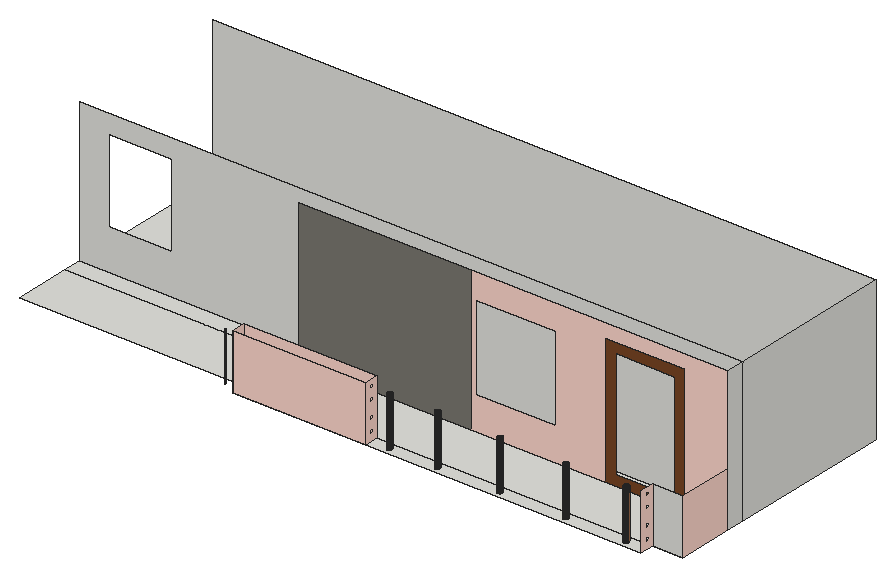
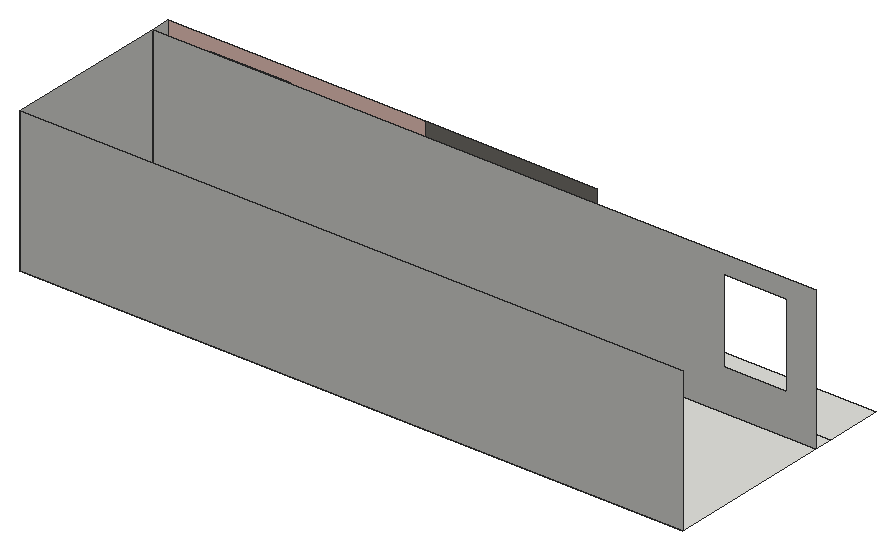
# SketchUp Ruby script. Lengths in inches.
U = 1.inch
M = Sketchup.active_model
def pt(a) = Geom::Point3d.new(a.map { |v| v * U })
def face(e, loops, mat)
  f = e.add_face(loops[0].map { |a| pt(a) })
  loops[1..].each { |l| e.add_face(l.map { |a| pt(a) }).erase! }
  f.material = f.back_material = mat if mat
  f
end
# faces: each face lists its corners as indices into pts; further lists are holes
def faces(e, pts, list, mat = nil) = list.each { |f| face(e, (f[0].is_a?(Array) ? f : [f]).map { |l| l.map { |i| pts[i] } }, mat) }
# xy, xz, yz: faces in a plane at the given z, y or x. An outline is a flat list of corners, or four numbers for a rectangle; further outlines are holes
def ring(l) = l.size == 4 ? [[l[0], l[1]], [l[2], l[1]], [l[2], l[3]], [l[0], l[3]]] : l.each_slice(2).to_a
def flat(e, list, mat, &to3) = list.each { |f| face(e, (f[0].is_a?(Array) ? f : [f]).map { |l| ring(l).map { |u, v| to3.(u, v) } }, mat) }
def xy(e, z, list, mat = nil) = flat(e, list, mat) { |x, y| [x, y, z] }
def xz(e, y, list, mat = nil) = flat(e, list, mat) { |x, z| [x, y, z] }
def yz(e, x, list, mat = nil) = flat(e, list, mat) { |y, z| [x, y, z] }
def lines(e, pts, list) = list.each { |a, b| e.add_line(pt(pts[a]), pt(pts[b])) }
# prism: a flat outline (further loops are holes) pulled along v
def prism(e, loops, v, mat = nil)
  f = face(e, loops, mat); d = Geom::Vector3d.new(v.map { |x| x * U })
  f.pushpull(f.normal.samedirection?(d) ? d.length : -d.length)
end
def box(e, o, s, mat = nil) = prism(e, [[o, [o[0] + s[0], o[1], o[2]], [o[0] + s[0], o[1] + s[1], o[2]], [o[0], o[1] + s[1], o[2]]]], [0, 0, s[2]], mat)
def at(x, y, z, deg = 0) = Geom::Transformation.translation(pt([x, y, z])) * Geom::Transformation.rotation(ORIGIN, Z_AXIS, deg.degrees)
def axes(o, x, y, z) = Geom::Transformation.new([*x, 0, *y, 0, *z, 0, *pt(o).to_a, 1])
def part(name) = M.definitions.add(name)
# library, detail: a bought-in or finely detailed component or shape, given as its bounding box
def library(name, o, s) = part(name).tap { |d| box(d.entities, o, s) }
def detail(e, o, s) = box(e.add_group.entities, o, s)
def put(e, d, t, mat = nil) = e.add_instance(d, t).tap { |i| i.material = mat if mat }
def group(e, t, mat = nil) = e.add_group.tap { |g| g.transformation = t; g.material = mat if mat }.entities
root = M.entities
M.materials.add("[Color B01]").color = [255, 216, 204]
M.materials.add("[Rough Square Concrete Block]").color = [123, 120, 113]
M.materials.add("[Wood Veneer 01]1").color = [120, 70, 37]
M.materials.add("[Wood Veneer 02]").color = [190, 128, 91]
xy(root,1956.4375,[[1053.15,267.5625,1631.4,328.8],[[1631.4,267.5625,2829.41,328.8],[1711.75,285.86,1709,286.22,1706.4375,287.28,1704.24,288.97,1702.55,291.17,1701.49,293.73,1701.125,296.48,1701.49,299.23,1702.55,301.79,1704.24,303.99,1706.4375,305.68,1709,306.74,1711.75,307.11,1714.5,306.74,1717.0625,305.68,1719.26,303.99,1720.95,301.79,1722.01,299.23,1722.375,296.48,1722.01,293.73,1720.95,291.17,1719.26,288.97,1717.0625,287.28,1714.5,286.22],[2741.25,285.86,2738.5,286.22,2735.9375,287.28,2733.74,288.97,2732.05,291.17,2730.99,293.73,2730.625,296.48,2730.99,299.23,2732.05,301.79,2733.74,303.99,2735.9375,305.68,2738.5,306.74,2741.25,307.11,2744,306.74,2746.5625,305.68,2748.76,303.99,2750.45,301.79,2751.51,299.23,2751.875,296.48,2751.51,293.73,2750.45,291.17,2748.76,288.97,2746.5625,287.28,2744,286.22],[1920.9375,285.86,1918.1875,286.22,1915.625,287.28,1913.42,288.97,1911.74,291.17,1910.67,293.73,1910.3125,296.48,1910.67,299.23,1911.74,301.79,1913.42,303.99,1915.625,305.68,1918.1875,306.74,1920.9375,307.11,1923.6875,306.74,1926.25,305.68,1928.45,303.99,1930.14,301.79,1931.2,299.23,1931.5625,296.48,1931.2,293.73,1930.14,291.17,1928.45,288.97,1926.25,287.28,1923.6875,286.22],[2479.625,285.86,2476.875,286.22,2474.3125,287.28,2472.11,288.97,2470.42,291.17,2469.36,293.73,2469,296.48,2469.36,299.23,2470.42,301.79,2472.11,303.99,2474.3125,305.68,2476.875,306.74,2479.625,307.11,2482.375,306.74,2484.9375,305.68,2487.14,303.99,2488.83,301.79,2489.89,299.23,2490.25,296.48,2489.89,293.73,2488.83,291.17,2487.14,288.97,2484.9375,287.28,2482.375,286.22],[2192.5,285.86,2189.75,286.22,2187.1875,287.28,2184.99,288.97,2183.3,291.17,2182.24,293.73,2181.875,296.48,2182.24,299.23,2183.3,301.79,2184.99,303.99,2187.1875,305.68,2189.75,306.74,2192.5,307.11,2195.25,306.74,2197.8125,305.68,2200.01,303.99,2201.7,301.79,2202.76,299.23,2203.125,296.48,2202.76,293.73,2201.7,291.17,2200.01,288.97,2197.8125,287.28,2195.25,286.22]],[1711.75,285.86,1709,286.22,1706.4375,287.28,1704.24,288.97,1702.55,291.17,1701.49,293.73,1701.125,296.48,1701.49,299.23,1702.55,301.79,1704.24,303.99,1706.4375,305.68,1709,306.74,1711.75,307.11,1714.5,306.74,1717.0625,305.68,1719.26,303.99,1720.95,301.79,1722.01,299.23,1722.375,296.48,1722.01,293.73,1720.95,291.17,1719.26,288.97,1717.0625,287.28,1714.5,286.22],[1920.9375,285.86,1918.1875,286.22,1915.625,287.28,1913.42,288.97,1911.74,291.17,1910.67,293.73,1910.3125,296.48,1910.67,299.23,1911.74,301.79,1913.42,303.99,1915.625,305.68,1918.1875,306.74,1920.9375,307.11,1923.6875,306.74,1926.25,305.68,1928.45,303.99,1930.14,301.79,1931.2,299.23,1931.5625,296.48,1931.2,293.73,1930.14,291.17,1928.45,288.97,1926.25,287.28,1923.6875,286.22],[2192.5,285.86,2189.75,286.22,2187.1875,287.28,2184.99,288.97,2183.3,291.17,2182.24,293.73,2181.875,296.48,2182.24,299.23,2183.3,301.79,2184.99,303.99,2187.1875,305.68,2189.75,306.74,2192.5,307.11,2195.25,306.74,2197.8125,305.68,2200.01,303.99,2201.7,301.79,2202.76,299.23,2203.125,296.48,2202.76,293.73,2201.7,291.17,2200.01,288.97,2197.8125,287.28,2195.25,286.22],
  [2479.625,285.86,2476.875,286.22,2474.3125,287.28,2472.11,288.97,2470.42,291.17,2469.36,293.73,2469,296.48,2469.36,299.23,2470.42,301.79,2472.11,303.99,2474.3125,305.68,2476.875,306.74,2479.625,307.11,2482.375,306.74,2484.9375,305.68,2487.14,303.99,2488.83,301.79,2489.89,299.23,2490.25,296.48,2489.89,293.73,2488.83,291.17,2487.14,288.97,2484.9375,287.28,2482.375,286.22],[2741.25,285.86,2738.5,286.22,2735.9375,287.28,2733.74,288.97,2732.05,291.17,2730.99,293.73,2730.625,296.48,2730.99,299.23,2732.05,301.79,2733.74,303.99,2735.9375,305.68,2738.5,306.74,2741.25,307.11,2744,306.74,2746.5625,305.68,2748.76,303.99,2750.45,301.79,2751.51,299.23,2751.875,296.48,2751.51,293.73,2750.45,291.17,2748.76,288.97,2746.5625,287.28,2744,286.22],[77.93,328.8,2962.22,571.9],[77.93,571.9,2962.22,653.97],[77.93,653.97,2962.22,1377.24]])
xz(root,267.5625,[[1053.15,1956.4375,1631.4,2195.8125]],"[Color B01]")
xz(root,328.8,[[2829.41,1956.4375,2962.22,2195.8125]])
xz(root,328.8,[[1053.15,1956.4375,1631.4,2195.8125]],"[Color B01]")
xz(root,571.9,[[[1845.89,1956.4375,2429.34,1956.4375,2429.34,2519.61,2777.4,2519.61,2777.4,1956.4375,2962.22,1956.4375,2962.22,2577.9375,1845.89,2577.9375],[1867.29,2101.11,2212.79,2469.24]]],"[Color B01]")
xz(root,571.9,[[1096.47,1956.4375,1845.89,2577.9375]],"[Rough Square Concrete Block]")
xz(root,571.9,[[[2429.34,1956.4375,2777.4,2519.61],[2473.97,2001.07,2732.77,2474.99]]],"[Wood Veneer 01]1")
xz(root,653.97,[[[77.93,1956.4375,2962.22,2577.9375],[206.78,2135.23,480.91,2496.04]]])
xz(root,1377.24,[[77.93,1956.4375,2962.22,2577.9375]])
yz(root,1053.15,[[[267.5625,1956.4375,328.8,2195.8125],[300.84,2164.31,302.34,2164.51,303.74,2165.09,304.95,2166.01,305.87,2167.21,306.45,2168.62,306.65,2170.12,306.45,2171.625,305.87,2173.03,304.95,2174.23,303.74,2175.15,302.34,2175.73,300.84,2175.93,299.33,2175.73,297.93,2175.15,296.73,2174.23,295.8,2173.03,295.22,2171.625,295.02,2170.12,295.22,2168.62,295.8,2167.21,296.73,2166.01,297.93,2165.09,299.33,2164.51],[300.84,1977.93,302.34,1978.13,303.74,1978.71,304.95,1979.63,305.87,1980.84,306.45,1982.24,306.65,1983.74,306.45,1985.25,305.87,1986.65,304.95,1987.85,303.74,1988.78,302.34,1989.36,300.84,1989.56,299.33,1989.36,297.93,1988.78,296.73,1987.85,295.8,1986.65,295.22,1985.25,295.02,1983.74,295.22,1982.24,295.8,1980.84,296.73,1979.63,297.93,1978.71,299.33,1978.13],[300.84,2119.12,302.34,2119.32,303.74,2119.9,304.95,2120.82,305.87,2122.03,306.45,2123.43,306.65,2124.93,306.45,2126.4375,305.87,2127.84,304.95,2129.04,303.74,2129.97,302.34,2130.55,300.84,2130.74,299.33,2130.55,297.93,2129.97,296.73,2129.04,295.8,2127.84,295.22,2126.4375,295.02,2124.93,295.22,2123.43,295.8,2122.03,296.73,2120.82,297.93,2119.9,299.33,2119.32],[300.84,2017.49,302.34,2017.69,303.74,2018.27,304.95,2019.2,305.87,2020.4,306.45,2021.8,306.65,2023.31,306.45,2024.8125,305.87,2026.21,304.95,2027.42,303.74,2028.34,302.34,2028.92,300.84,2029.12,299.33,2028.92,297.93,2028.34,296.73,2027.42,295.8,2026.21,295.22,2024.8125,295.02,2023.31,295.22,2021.8,295.8,2020.4,296.73,2019.2,297.93,2018.27,299.33,2017.69],[300.84,2076.99,302.34,2077.19,303.74,2077.77,304.95,2078.7,305.87,2079.9,306.45,2081.3,306.65,2082.81,306.45,2084.3125,305.87,2085.71,304.95,2086.92,303.74,2087.84,302.34,2088.42,300.84,2088.62,299.33,2088.42,297.93,2087.84,296.73,2086.92,295.8,2085.71,295.22,2084.3125,295.02,2082.81,295.22,2081.3,295.8,2079.9,296.73,2078.7,297.93,2077.77,299.33,2077.19]]],"[Color B01]")
yz(root,1631.4,[[[267.5625,1956.4375,328.8,2195.8125],[299.17,2162.9,296.83,2163.21,294.64,2164.12,292.77,2165.56,291.33,2167.43,290.42,2169.62,290.11,2171.97,290.42,2174.3125,291.33,2176.5,292.77,2178.375,294.64,2179.8125,296.83,2180.72,299.17,2181.03,301.52,2180.72,303.71,2179.8125,305.58,2178.375,307.02,2176.5,307.93,2174.3125,308.24,2171.97,307.93,2169.62,307.02,2167.43,305.58,2165.56,303.71,2164.12,301.52,2163.21],[299.17,2111.15,296.83,2111.46,294.64,2112.37,292.77,2113.81,291.33,2115.68,290.42,2117.87,290.11,2120.22,290.42,2122.5625,291.33,2124.75,292.77,2126.625,294.64,2128.0625,296.83,2128.97,299.17,2129.28,301.52,2128.97,303.71,2128.0625,305.58,2126.625,307.02,2124.75,307.93,2122.5625,308.24,2120.22,307.93,2117.87,307.02,2115.68,305.58,2113.81,303.71,2112.37,301.52,2111.46],[299.17,2040.72,296.83,2041.02,294.64,2041.93,292.77,2043.37,291.33,2045.25,290.42,2047.43,290.11,2049.78,290.42,2052.125,291.33,2054.31,292.77,2056.1875,294.64,2057.625,296.83,2058.53,299.17,2058.84,301.52,2058.53,303.71,2057.625,305.58,2056.1875,307.02,2054.31,307.93,2052.125,308.24,2049.78,307.93,2047.43,307.02,2045.25,305.58,2043.37,303.71,2041.93,301.52,2041.02],[299.17,1985.65,296.83,1985.96,294.64,1986.87,292.77,1988.31,291.33,1990.18,290.42,1992.37,290.11,1994.72,290.42,1997.0625,291.33,1999.25,292.77,2001.125,294.64,2002.5625,296.83,2003.47,299.17,2003.78,301.52,2003.47,303.71,2002.5625,305.58,2001.125,307.02,1999.25,307.93,1997.0625,308.24,1994.72,307.93,1992.37,307.02,1990.18,305.58,1988.31,303.71,1986.87,301.52,1985.96]]],"[Color B01]")
yz(root,2829.41,[[[267.5625,1956.4375,328.8,2195.8125],[299.17,2162.9,301.52,2163.21,303.71,2164.12,305.58,2165.56,307.02,2167.43,307.93,2169.62,308.24,2171.97,307.93,2174.3125,307.02,2176.5,305.58,2178.375,303.71,2179.8125,301.52,2180.72,299.17,2181.03,296.83,2180.72,294.64,2179.8125,292.77,2178.375,291.33,2176.5,290.42,2174.3125,290.11,2171.97,290.42,2169.62,291.33,2167.43,292.77,2165.56,294.64,2164.12,296.83,2163.21],[299.17,1985.65,301.52,1985.96,303.71,1986.87,305.58,1988.31,307.02,1990.18,307.93,1992.37,308.24,1994.72,307.93,1997.0625,307.02,1999.25,305.58,2001.125,303.71,2002.5625,301.52,2003.47,299.17,2003.78,296.83,2003.47,294.64,2002.5625,292.77,2001.125,291.33,1999.25,290.42,1997.0625,290.11,1994.72,290.42,1992.37,291.33,1990.18,292.77,1988.31,294.64,1986.87,296.83,1985.96],[299.17,2111.15,301.52,2111.46,303.71,2112.37,305.58,2113.81,307.02,2115.68,307.93,2117.87,308.24,2120.22,307.93,2122.5625,307.02,2124.75,305.58,2126.625,303.71,2128.0625,301.52,2128.97,299.17,2129.28,296.83,2128.97,294.64,2128.0625,292.77,2126.625,291.33,2124.75,290.42,2122.5625,290.11,2120.22,290.42,2117.87,291.33,2115.68,292.77,2113.81,294.64,2112.37,296.83,2111.46],[299.17,2040.72,301.52,2041.02,303.71,2041.93,305.58,2043.37,307.02,2045.25,307.93,2047.43,308.24,2049.78,307.93,2052.125,307.02,2054.31,305.58,2056.1875,303.71,2057.625,301.52,2058.53,299.17,2058.84,296.83,2058.53,294.64,2057.625,292.77,2056.1875,291.33,2054.31,290.42,2052.125,290.11,2049.78,290.42,2047.43,291.33,2045.25,292.77,2043.37,294.64,2041.93,296.83,2041.02]]],"[Color B01]")
yz(root,2962.22,[[571.9,1956.4375,653.97,2577.9375],[653.97,1956.4375,1377.24,2577.9375]])
yz(root,2962.22,[[328.8,1956.4375,571.9,2195.8125]],"[Color B01]")
p = [[1709,286.22,1956.4375],[1711.75,285.86,1956.4375],[1711.75,285.86,2171.4375],[1709,286.22,2171.4375],[1714.5,286.22,1956.4375],[1714.5,286.22,2171.4375],
  [1918.1875,286.22,1956.4375],[1920.9375,285.86,1956.4375],[1920.9375,285.86,2176.5],[1918.1875,286.22,2176.5],[1923.6875,286.22,1956.4375],[1923.6875,286.22,2176.5],
  [2189.75,286.22,1956.4375],[2192.5,285.86,1956.4375],[2192.5,285.86,2169.6875],[2189.75,286.22,2169.6875],[2195.25,286.22,1956.4375],[2195.25,286.22,2169.6875],
  [2476.875,286.22,1956.4375],[2479.625,285.86,1956.4375],[2479.625,285.86,2168.9375],[2476.875,286.22,2168.9375],[2482.375,286.22,1956.4375],[2482.375,286.22,2168.9375],
  [2738.5,286.22,1956.4375],[2741.25,285.86,1956.4375],[2741.25,285.86,2173.25],[2738.5,286.22,2173.25],[2744,286.22,1956.4375],[2744,286.22,2173.25],
  [1706.4375,287.28,1956.4375],[1706.4375,287.28,2171.4375],[1717.0625,287.28,1956.4375],[1717.0625,287.28,2171.4375],[1915.625,287.28,1956.4375],[1915.625,287.28,2176.5],
  [1926.25,287.28,1956.4375],[1926.25,287.28,2176.5],[2187.1875,287.28,1956.4375],[2187.1875,287.28,2169.6875],[2197.8125,287.28,1956.4375],[2197.8125,287.28,2169.6875],
  [2474.3125,287.28,1956.4375],[2474.3125,287.28,2168.9375],[2484.9375,287.28,1956.4375],[2484.9375,287.28,2168.9375],[2735.9375,287.28,1956.4375],[2735.9375,287.28,2173.25],
  [2746.5625,287.28,1956.4375],[2746.5625,287.28,2173.25],[1704.24,288.97,1956.4375],[1704.24,288.97,2171.4375],[1719.26,288.97,1956.4375],[1719.26,288.97,2171.4375],
  [1913.42,288.97,1956.4375],[1913.42,288.97,2176.5],[1928.45,288.97,1956.4375],[1928.45,288.97,2176.5],[2184.99,288.97,1956.4375],[2184.99,288.97,2169.6875],
  [2200.01,288.97,1956.4375],[2200.01,288.97,2169.6875],[2472.11,288.97,1956.4375],[2472.11,288.97,2168.9375],[2487.14,288.97,1956.4375],[2487.14,288.97,2168.9375],
  [2733.74,288.97,1956.4375],[2733.74,288.97,2173.25],[2748.76,288.97,1956.4375],[2748.76,288.97,2173.25],[1702.55,291.17,1956.4375],[1702.55,291.17,2171.4375],
  [1720.95,291.17,1956.4375],[1720.95,291.17,2171.4375],[1911.74,291.17,1956.4375],[1911.74,291.17,2176.5],[1930.14,291.17,1956.4375],[1930.14,291.17,2176.5],
  [2183.3,291.17,1956.4375],[2183.3,291.17,2169.6875],[2201.7,291.17,1956.4375],[2201.7,291.17,2169.6875],[2470.42,291.17,1956.4375],[2470.42,291.17,2168.9375],
  [2488.83,291.17,1956.4375],[2488.83,291.17,2168.9375],[2732.05,291.17,1956.4375],[2732.05,291.17,2173.25],[2750.45,291.17,1956.4375],[2750.45,291.17,2173.25],
  [1701.49,293.73,1956.4375],[1701.49,293.73,2171.4375],[1722.01,293.73,1956.4375],[1722.01,293.73,2171.4375],[1910.67,293.73,1956.4375],[1911.67,291.33,2176.5],
  [1910.67,293.73,2176.5],[1931.2,293.73,1956.4375],[1931.2,293.73,2176.5],[1930.2,291.33,2176.5],[2182.24,293.73,1956.4375],[2182.24,293.73,2169.6875],
  [2202.76,293.73,1956.4375],[2202.76,293.73,2169.6875],[2469.36,293.73,1956.4375],[2469.36,293.73,2168.9375],[2489.89,293.73,1956.4375],[2489.89,293.73,2168.9375],
  [2730.99,293.73,1956.4375],[2730.99,293.73,2173.25],[2751.51,293.73,1956.4375],[2751.51,293.73,2173.25],[1701.125,296.48,1956.4375],[1701.125,296.48,2171.4375],
  [1722.375,296.48,1956.4375],[1722.375,296.48,2171.4375],[1910.3125,296.48,1956.4375],[1910.3125,296.48,2176.5],[1931.5625,296.48,1956.4375],[1931.5625,296.48,2176.5],
  [2181.875,296.48,1956.4375],[2181.875,296.48,2169.6875],[2203.125,296.48,1956.4375],[2203.125,296.48,2169.6875],[2469,296.48,1956.4375],[2469,296.48,2168.9375],
  [2490.25,296.48,1956.4375],[2490.25,296.48,2168.9375],[2730.625,296.48,1956.4375],[2730.625,296.48,2173.25],[2751.875,296.48,1956.4375],[2751.875,296.48,2173.25],
  [1701.49,299.23,1956.4375],[1701.49,299.23,2171.4375],[1722.01,299.23,1956.4375],[1722.01,299.23,2171.4375],[1910.67,299.23,1956.4375],[1910.67,299.23,2176.5],
  [1931.2,299.23,1956.4375],[1931.2,299.23,2176.5],[2182.24,299.23,1956.4375],[2182.24,299.23,2169.6875],[2202.76,299.23,1956.4375],[2202.76,299.23,2169.6875],
  [2469.36,299.23,1956.4375],[2469.36,299.23,2168.9375],[2489.89,299.23,1956.4375],[2489.89,299.23,2168.9375],[2730.99,299.23,1956.4375],[2730.99,299.23,2173.25],
  [2751.51,299.23,1956.4375],[2751.51,299.23,2173.25],[995.5,296.85,1956.4375],[995.77,298.86,1956.4375],[995.77,298.86,2170.12],[995.5,296.85,2170.12],
  [995.5,300.86,1956.4375],[995.5,300.86,2170.12],[1702.55,301.79,1956.4375],[1702.55,301.79,2171.4375],[1720.95,301.79,1956.4375],[1720.95,301.79,2171.4375],
  [1911.74,301.79,1956.4375],[1911.74,301.79,2176.5],[1930.14,301.79,1956.4375],[1930.14,301.79,2176.5],[2183.3,301.79,1956.4375],[2183.3,301.79,2169.6875],
  [2201.7,301.79,1956.4375],[2201.7,301.79,2169.6875],[2470.42,301.79,1956.4375],[2470.42,301.79,2168.9375],[2488.83,301.79,1956.4375],[2488.83,301.79,2168.9375],
  [2732.05,301.79,1956.4375],[2732.05,301.79,2173.25],[2750.45,301.79,1956.4375],[2750.45,301.79,2173.25],[1704.24,303.99,1956.4375],[1704.24,303.99,2171.4375],
  [1719.26,303.99,1956.4375],[1719.26,303.99,2171.4375],[1913.42,303.99,1956.4375],[1913.42,303.99,2176.5],[1928.45,303.99,1956.4375],[1928.45,303.99,2176.5],
  [2184.99,303.99,1956.4375],[2184.99,303.99,2169.6875],[2200.01,303.99,1956.4375],[2200.01,303.99,2169.6875],[2472.11,303.99,1956.4375],[2472.11,303.99,2168.9375],
  [2487.14,303.99,1956.4375],[2487.14,303.99,2168.9375],[2733.74,303.99,1956.4375],[2733.74,303.99,2173.25],[2748.76,303.99,1956.4375],[2748.76,303.99,2173.25],
  [1706.4375,305.68,1956.4375],[1706.4375,305.68,2171.4375],[1717.0625,305.68,1956.4375],[1717.0625,305.68,2171.4375],[1915.625,305.68,1956.4375],[1915.625,305.68,2176.5],
  [1926.25,305.68,1956.4375],[1926.25,305.68,2176.5],[2187.1875,305.68,1956.4375],[2187.1875,305.68,2169.6875],[2197.8125,305.68,1956.4375],[2197.8125,305.68,2169.6875],
  [2474.3125,305.68,1956.4375],[2474.3125,305.68,2168.9375],[2484.9375,305.68,1956.4375],[2484.9375,305.68,2168.9375],[2735.9375,305.68,1956.4375],[2735.9375,305.68,2173.25],
  [2746.5625,305.68,1956.4375],[2746.5625,305.68,2173.25],[1709,306.74,1956.4375],[1709,306.74,2171.4375],[1714.5,306.74,1956.4375],[1714.5,306.74,2171.4375],
  [1918.1875,306.74,1956.4375],[1918.1875,306.74,2176.5],[1923.6875,306.74,1956.4375],[1923.6875,306.74,2176.5],[2189.75,306.74,1956.4375],[2189.75,306.74,2169.6875],
  [2195.25,306.74,1956.4375],[2195.25,306.74,2169.6875],[2476.875,306.74,1956.4375],[2476.875,306.74,2168.9375],[2482.375,306.74,1956.4375],[2482.375,306.74,2168.9375],
  [2738.5,306.74,1956.4375],[2738.5,306.74,2173.25],[2744,306.74,1956.4375],[2744,306.74,2173.25],[1711.75,307.11,1956.4375],[1711.75,307.11,2171.4375],
  [1920.9375,307.11,1956.4375],[1920.3125,307.02,2176.5],[1920.9375,307.11,2176.5],[1921.5625,307.02,2176.5],[2192.5,307.11,1956.4375],[2192.5,307.11,2169.6875],
  [2479.625,307.11,1956.4375],[2479.625,307.11,2168.9375],[2741.25,307.11,1956.4375],[2741.25,307.11,2173.25]]
faces(root,p,[[0,1,2,3],[1,4,5,2],[6,7,8,9],[7,10,11,8],[12,13,14,15],[13,16,17,14],[18,19,20,21],[19,22,23,20],
  [24,25,26,27],[25,28,29,26],[30,0,3,31],[4,32,33,5],[34,6,9,35],[10,36,37,11],[38,12,15,39],[16,40,41,17],
  [42,18,21,43],[22,44,45,23],[46,24,27,47],[28,48,49,29],[50,30,31,51],[32,52,53,33],[54,34,35,55],[36,56,57,37],
  [58,38,39,59],[40,60,61,41],[62,42,43,63],[44,64,65,45],[66,46,47,67],[48,68,69,49],[70,50,51,71],[52,72,73,53],
  [74,54,55,75],[56,76,77,57],[78,58,59,79],[60,80,81,61],[82,62,63,83],[64,84,85,65],[86,66,67,87],[68,88,89,69],
  [90,70,71,91],[72,92,93,73],[94,74,75,95,96],[76,97,98,99,77],[100,78,79,101],[80,102,103,81],[104,82,83,105],[84,106,107,85],
  [108,86,87,109],[88,110,111,89],[112,90,91,113],[92,114,115,93],[116,94,96,117],[97,118,119,98],[120,100,101,121],[102,122,123,103],
  [124,104,105,125],[106,126,127,107],[128,108,109,129],[110,130,131,111],[132,112,113,133],[114,134,135,115],[136,116,117,137],[118,138,139,119],
  [140,120,121,141],[122,142,143,123],[144,124,125,145],[126,146,147,127],[148,128,129,149],[130,150,151,131],[152,153,154,155],[153,156,157,154],
  [158,132,133,159],[134,160,161,135],[162,136,137,163],[138,164,165,139],[166,140,141,167],[142,168,169,143],[170,144,145,171],[146,172,173,147],
  [174,148,149,175],[150,176,177,151],[178,158,159,179],[160,180,181,161],[182,162,163,183],[164,184,185,165],[186,166,167,187],[168,188,189,169],
  [190,170,171,191],[172,192,193,173],[194,174,175,195],[176,196,197,177],[198,178,179,199],[180,200,201,181],[202,182,183,203],[184,204,205,185],
  [206,186,187,207],[188,208,209,189],[210,190,191,211],[192,212,213,193],[214,194,195,215],[196,216,217,197],[218,198,199,219],[200,220,221,201],
  [222,202,203,223],[204,224,225,205],[226,206,207,227],[208,228,229,209],[230,210,211,231],[212,232,233,213],[234,214,215,235],[216,236,237,217],
  [238,218,219,239],[220,238,239,221],[240,222,223,241,242],[224,240,242,243,225],[244,226,227,245],[228,244,245,229],[246,230,231,247],[232,246,247,233],
  [248,234,235,249],[236,248,249,237]],"[Wood Veneer 02]")
